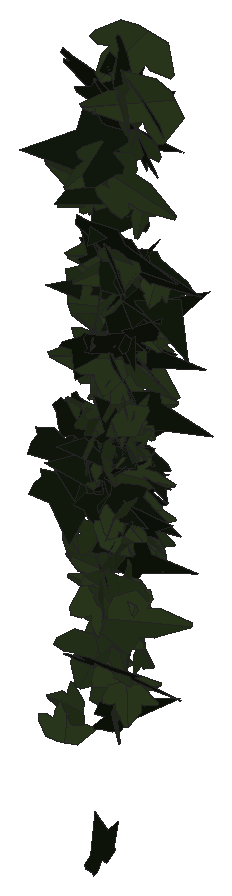
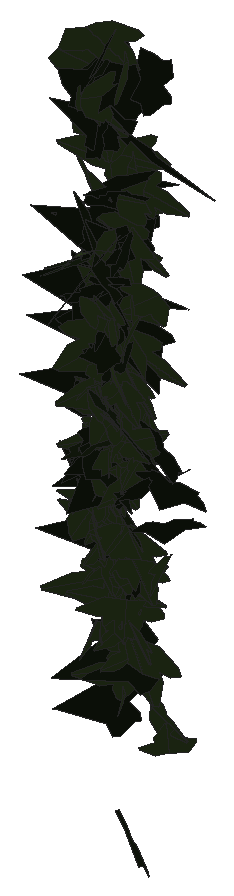
# SketchUp Ruby script. Lengths in inches.
U = 1.inch
M = Sketchup.active_model
def pt(a) = Geom::Point3d.new(a.map { |v| v * U })
def face(e, loops, mat)
  f = e.add_face(loops[0].map { |a| pt(a) })
  loops[1..].each { |l| e.add_face(l.map { |a| pt(a) }).erase! }
  f.material = f.back_material = mat if mat
  f
end
# faces: each face lists its corners as indices into pts; further lists are holes
def faces(e, pts, list, mat = nil) = list.each { |f| face(e, (f[0].is_a?(Array) ? f : [f]).map { |l| l.map { |i| pts[i] } }, mat) }
# xy, xz, yz: faces in a plane at the given z, y or x. An outline is a flat list of corners, or four numbers for a rectangle; further outlines are holes
def ring(l) = l.size == 4 ? [[l[0], l[1]], [l[2], l[1]], [l[2], l[3]], [l[0], l[3]]] : l.each_slice(2).to_a
def flat(e, list, mat, &to3) = list.each { |f| face(e, (f[0].is_a?(Array) ? f : [f]).map { |l| ring(l).map { |u, v| to3.(u, v) } }, mat) }
def xy(e, z, list, mat = nil) = flat(e, list, mat) { |x, y| [x, y, z] }
def xz(e, y, list, mat = nil) = flat(e, list, mat) { |x, z| [x, y, z] }
def yz(e, x, list, mat = nil) = flat(e, list, mat) { |y, z| [x, y, z] }
def lines(e, pts, list) = list.each { |a, b| e.add_line(pt(pts[a]), pt(pts[b])) }
# prism: a flat outline (further loops are holes) pulled along v
def prism(e, loops, v, mat = nil)
  f = face(e, loops, mat); d = Geom::Vector3d.new(v.map { |x| x * U })
  f.pushpull(f.normal.samedirection?(d) ? d.length : -d.length)
end
def box(e, o, s, mat = nil) = prism(e, [[o, [o[0] + s[0], o[1], o[2]], [o[0] + s[0], o[1] + s[1], o[2]], [o[0], o[1] + s[1], o[2]]]], [0, 0, s[2]], mat)
def at(x, y, z, deg = 0) = Geom::Transformation.translation(pt([x, y, z])) * Geom::Transformation.rotation(ORIGIN, Z_AXIS, deg.degrees)
def axes(o, x, y, z) = Geom::Transformation.new([*x, 0, *y, 0, *z, 0, *pt(o).to_a, 1])
def part(name) = M.definitions.add(name)
# library, detail: a bought-in or finely detailed component or shape, given as its bounding box
def library(name, o, s) = part(name).tap { |d| box(d.entities, o, s) }
def detail(e, o, s) = box(e.add_group.entities, o, s)
def put(e, d, t, mat = nil) = e.add_instance(d, t).tap { |i| i.material = mat if mat }
def group(e, t, mat = nil) = e.add_group.tap { |g| g.transformation = t; g.material = mat if mat }.entities
root = M.entities
M.materials.add("1026 AP 7946 SUNNY SIDE UP").color = [254, 231, 186]
M.materials.add("efeu1").color = [18, 25, 13]
M.materials.add("efeu2").color = [43, 57, 29]
c1 = part("ivyleaf_10")
p = [[0,0.5,-0.03],[-0.0625,2.02,-0.43],[-0.19,2.01,-0.46],[-0.54,1.05,-0.29],[-0.52,0.625,-0.18],[-0.83,0.76,-0.28],
  [-1.16,0.64,-0.33],[-1.15,0.33,-0.24],[-0.77,-0.39,0.02],[-0.3,-0.51,0.16],[0.04,-0.48,0.23],[-0.02,2.01,-0.4375],
  [-0.06,2.01,-0.43],[0.04,-0.49,0.23],[0.67,-0.49,0.14],[1.38,0.36,-0.2],[1.375,0.51,-0.24],[0.81,0.65,-0.19],
  [0.62,0.59,-0.15],[0.6,1.09,-0.28],[0.5,1.23,-0.31]]
faces(c1.entities,p,[[0,1,2,3,4,5,6,7,8,9,10],[11,12,0,13,14,15,16,17,18,19,20]],"efeu2")
c2 = part("ivyleaf_9")
p = [[1.54,2.16,1.25],[1.36,2.04,1.19],[-0.21,0.99,0.68],[-0.71,1.11,0.82],[-0.85,0.86,0.67],[-0.8,0.17,0.21],
  [-0.9,-0.01,0.1],[-0.67,-0.16,-0.02],[-0.08,-0.08,-0.05],[-0.03,-0.6,-0.4],[0.65,-0.88,-0.66],[0.83,-0.6,-0.49],
  [1.29,-0.42,-0.43],[1.8125,-0.07,-0.26],[1.21,0.44,0.15]]
faces(c2.entities,p,[[0,1,2,3,4,5,6,7,8,9,10,11,12,13,14]],"efeu1")
put(root,c1,axes([137.62,209.9,263.875],[0.11766,-0.06862,-0.22002],[0.29984,-0.09834,0.10099],[-0.18465,-0.2034,0.0238]),"1026 AP 7946 SUNNY SIDE UP")
put(root,c1,axes([138.34,209.98,262.02],[-0.01304,-0.02369,-0.22765],[0.16421,-0.19546,0.01642],[-0.30824,-0.10313,0.01838]),"1026 AP 7946 SUNNY SIDE UP")
put(root,c2,axes([138.23,209.71,261.3],[0.02182,-0.02112,-0.28857],[0.17202,0.25859,-0.01299],[0.40662,-0.10826,0.02098]),"1026 AP 7946 SUNNY SIDE UP")
put(root,c1,axes([138.18,209.91,258.03],[-0.11608,0.13996,-0.13331],[0.0679,-0.12375,-0.16299],[-0.2928,-0.08418,0.01505]),"1026 AP 7946 SUNNY SIDE UP")
put(root,c1,axes([137.95,210,266.1],[0.15276,0.12837,-0.25399],[-0.19782,-0.21344,-0.16632],[-0.39088,0.15819,-0.01509]),"1026 AP 7946 SUNNY SIDE UP")
put(root,c1,axes([138.28,209.68,261.9],[-0.08528,0.14601,0.20223],[-0.11746,0.18069,-0.15934],[-0.36522,-0.09221,0.00403]),"1026 AP 7946 SUNNY SIDE UP")
put(root,c1,axes([138.4375,209.86,258.39],[0.2544,0.13602,-0.00184],[0.01288,-0.0137,-0.21723],[-0.21353,0.16123,-0.01529]),"1026 AP 7946 SUNNY SIDE UP")
put(root,c2,axes([137.89,209.875,264.94],[0.34828,-0.08327,0.22073],[0.29953,-0.10121,-0.24345],[0.20355,0.29142,-0.01943]),"1026 AP 7946 SUNNY SIDE UP")
put(root,c2,axes([138.25,209.86,263.39],[0.43405,0.17022,0.04183],[-0.07626,0.00341,0.33286],[0.26403,-0.27885,0.02737]),"1026 AP 7946 SUNNY SIDE UP")
put(root,c1,axes([138.28,209.8,262.375],[0.43233,0.00207,0.1601],[-0.24322,0.03423,0.28167],[-0.02366,-0.31396,0.02991]),"1026 AP 7946 SUNNY SIDE UP")
put(root,c1,axes([138.3125,209.87,259.98],[-0.37139,-0.04498,0.01945],[-0.02256,-0.02646,-0.24669],[0.07348,-0.23548,0.02256]),"1026 AP 7946 SUNNY SIDE UP")
put(root,c1,axes([138.22,209.9,263.73],[-0.36976,-0.11445,-0.01028],[-0.02652,0.0134,0.26876],[-0.17859,0.23496,-0.01863]),"1026 AP 7946 SUNNY SIDE UP")
put(root,c2,axes([138.03,209.86,263.46],[0.12723,0.19476,-0.17816],[-0.08352,-0.16613,-0.21793],[-0.40213,0.09612,-0.01111]),"1026 AP 7946 SUNNY SIDE UP")
put(root,c1,axes([137.65,209.82,257.88],[-0.03585,0.04062,0.21877],[-0.3322,0.04013,-0.03107],[-0.07057,-0.20954,0.03514]),"1026 AP 7946 SUNNY SIDE UP")
put(root,c1,axes([138.34,209.99,262.51],[0.22732,-0.12361,0.12794],[0.12629,-0.09736,-0.19563],[0.24575,0.16438,-0.01781]),"1026 AP 7946 SUNNY SIDE UP")
put(root,c1,axes([138.04,209.9,259.81],[-0.03934,0.20759,-0.05095],[-0.03372,-0.05316,-0.21393],[-0.33429,-0.01907,0.02757]),"1026 AP 7946 SUNNY SIDE UP")
put(root,c1,axes([138.36,209.78,261.08],[0.12975,0.2141,0.14012],[0.07645,0.12573,-0.23564],[-0.39041,0.09578,0.00042]),"1026 AP 7946 SUNNY SIDE UP")
put(root,c1,axes([138.25,209.8,260.95],[0.06837,-0.1428,-0.14948],[-0.02841,0.14425,-0.15184],[0.31794,0.0436,0.01858]),"1026 AP 7946 SUNNY SIDE UP")
put(root,c1,axes([138.27,209.85,260.4],[-0.01717,-0.19277,-0.08617],[0.02222,0.0818,-0.19822],[0.32898,-0.01559,0.00889]),"1026 AP 7946 SUNNY SIDE UP")
put(root,c2,axes([138.35,209.95,260.96],[0.34035,-0.0054,-0.13599],[0.20697,0.02982,0.22132],[0.01722,-0.25175,0.02764]),"1026 AP 7946 SUNNY SIDE UP")
put(root,c1,axes([138.39,209.78,260.64],[0.1623,0.23022,-0.11099],[0.05265,0.10437,0.26027],[0.39707,-0.10794,0.01085]),"1026 AP 7946 SUNNY SIDE UP")
put(root,c1,axes([137.4375,209.82,257.46],[0.23002,0.16719,-0.0549],[0.03486,0.05245,0.22847],[0.27417,-0.14694,0.01701]),"1026 AP 7946 SUNNY SIDE UP")
put(root,c1,axes([138.26,210.07,264.625],[0.11058,0.08861,-0.29481],[-0.29876,-0.21474,-0.11765],[-0.36516,0.20252,0.00698]),"1026 AP 7946 SUNNY SIDE UP")
put(root,c1,axes([138.27,209.99,261.29],[-0.19135,-0.18041,0.12846],[-0.09051,-0.11254,-0.22443],[0.3337,-0.13397,0.01279]),"1026 AP 7946 SUNNY SIDE UP")
put(root,c1,axes([138.07,209.89,263.22],[0.22008,-0.0723,-0.28753],[-0.42865,0.06643,-0.15841],[0.14567,0.30471,-0.03172]),"1026 AP 7946 SUNNY SIDE UP")
put(root,c2,axes([138.45,210,262.16],[0.14585,0.0591,0.25072],[-0.36132,-0.08224,0.11047],[0.15533,-0.24679,0.02155]),"1026 AP 7946 SUNNY SIDE UP")
put(root,c1,axes([137.98,209.86,262.15],[-0.04842,-0.20496,0.10238],[0.01741,0.1,0.21407],[-0.35855,0.03253,-0.00343]),"1026 AP 7946 SUNNY SIDE UP")
put(root,c1,axes([138.1,210.02,267.41],[-0.22712,0.22157,-0.23308],[0.15552,-0.20612,-0.27269],[-0.47452,-0.1736,0.02219]),"1026 AP 7946 SUNNY SIDE UP")
put(root,c1,axes([138.8125,209.99,267.26],[0.27411,-0.00345,-0.33382],[-0.50519,-0.04968,-0.17782],[-0.06625,0.36457,-0.02522]),"1026 AP 7946 SUNNY SIDE UP")
put(root,c1,axes([138.3,209.89,264.85],[0.26794,-0.0938,-0.27633],[-0.40019,0.08733,-0.19791],[0.19693,0.30508,-0.02621]),"1026 AP 7946 SUNNY SIDE UP")
put(root,c2,axes([138.39,209.9,261.96],[-0.3289,0.14447,0.11019],[-0.16399,0.03459,-0.26004],[-0.22926,-0.23199,0.02793]),"1026 AP 7946 SUNNY SIDE UP")
put(root,c1,axes([137.86,210.09,265.48],[-0.03464,-0.0343,0.24621],[-0.13683,-0.22294,-0.0425],[0.35446,-0.08942,0.00766]),"1026 AP 7946 SUNNY SIDE UP")
put(root,c1,axes([138.48,209.73,259.5625],[-0.05382,-0.07102,-0.35717],[0.41431,0.22682,-0.07342],[0.37057,-0.26391,0.03021]),"1026 AP 7946 SUNNY SIDE UP")
put(root,c1,axes([138.13,209.92,262.52],[-0.30391,0.08898,-0.04726],[0.05561,-0.03379,-0.21881],[-0.14766,-0.19587,0.01486]),"1026 AP 7946 SUNNY SIDE UP")
put(root,c1,axes([138.46,209.82,261.68],[-0.09617,-0.05671,-0.23973],[0.31171,0.12221,-0.08376],[0.21049,-0.20689,0.01451]),"1026 AP 7946 SUNNY SIDE UP")
put(root,c1,axes([138.12,209.95,265.9],[0.08261,0.03072,0.37081],[0.56592,0.02478,-0.05618],[-0.04566,0.36274,-0.02542]),"1026 AP 7946 SUNNY SIDE UP")
put(root,c2,axes([138.22,209.99,264.74],[0.26101,-0.1018,0.26469],[0.3372,-0.14267,-0.20135],[0.27544,0.27112,-0.00432]),"1026 AP 7946 SUNNY SIDE UP")
put(root,c2,axes([137.89,209.79,258.68],[0.51816,-0.00778,0.08323],[0.12585,0.08835,-0.32684],[-0.02163,0.3276,0.09218]),"1026 AP 7946 SUNNY SIDE UP")
put(root,c2,axes([137.85,210.09,259.77],[-0.03768,-0.00594,0.24814],[0.02936,-0.24141,-0.00563],[0.37778,0.01817,0.02519]),"1026 AP 7946 SUNNY SIDE UP")
put(root,c1,axes([138.44,210.09,259.84],[-0.15714,-0.09343,0.15565],[0.15159,-0.17457,-0.04637],[0.23546,0.05003,0.13373]),"1026 AP 7946 SUNNY SIDE UP")
put(root,c1,axes([138.54,209.9,261.23],[-0.07983,-0.20533,-0.07381],[0.03525,0.06704,-0.21744],[0.33953,-0.05523,0.00522]),"1026 AP 7946 SUNNY SIDE UP")
put(root,c2,axes([138.31,209.77,260.71],[-0.08724,0.18956,0.18302],[-0.08976,0.1672,-0.20241],[-0.39734,-0.07939,0.00554]),"1026 AP 7946 SUNNY SIDE UP")
put(root,c1,axes([138.34,209.8125,259.3],[-0.06909,-0.0426,0.23517],[0.18638,0.19596,0.06226],[-0.31443,0.12551,-0.01477]),"1026 AP 7946 SUNNY SIDE UP")
put(root,c1,axes([138.17,210.05,260.75],[-0.15109,0.04966,-0.20345],[0.16456,-0.17563,-0.09884],[-0.27518,-0.13229,0.0526]),"1026 AP 7946 SUNNY SIDE UP")
put(root,c2,axes([138.08,209.94,266.27],[-0.42862,0.15289,0.1432],[-0.21515,0.03697,-0.32009],[-0.24225,-0.30335,0.03091]),"1026 AP 7946 SUNNY SIDE UP")
put(root,c2,axes([137.99,210.05,261.88],[-0.36049,-0.03909,-0.20502],[0.31525,-0.00058,-0.23808],[0.04583,-0.30344,0.02506]),"1026 AP 7946 SUNNY SIDE UP")
put(root,c1,axes([137.79,210.17,263.78],[-0.01479,0.13256,-0.33305],[0.04231,-0.32292,-0.13879],[-0.54888,-0.02846,-0.00172]),"1026 AP 7946 SUNNY SIDE UP")
put(root,c1,axes([138.32,210.03,259.125],[0.03956,-0.21025,0.07734],[0.11555,-0.06472,-0.20915],[0.33215,0.04756,0.06354]),"1026 AP 7946 SUNNY SIDE UP")
put(root,c1,axes([138.39,210.11,262.46],[0.00989,-0.16493,0.18574],[0.01953,-0.18085,-0.17105],[0.38482,0.01341,0.00391]),"1026 AP 7946 SUNNY SIDE UP")
put(root,c1,axes([137.87,209.9375,258.79],[0.51065,-0.0235,-0.08446],[-0.11609,0.08313,-0.32587],[0.06673,0.32443,0.07942]),"1026 AP 7946 SUNNY SIDE UP")
put(root,c2,axes([137.45,210.01,267.31],[0.3407,-0.12689,0.12004],[0.13743,-0.0817,-0.25798],[0.23432,0.23242,-0.02322]),"1026 AP 7946 SUNNY SIDE UP")
put(root,c1,axes([138.27,209.95,261.98],[-0.25696,-0.0733,0.13413],[0.17874,0.06519,0.18458],[-0.15336,0.19879,-0.00962]),"1026 AP 7946 SUNNY SIDE UP")
put(root,c1,axes([138.31,209.93,264.02],[0.2704,0.11295,0.193],[0.27766,0.06761,-0.2093],[-0.20156,0.24466,-0.02941]),"1026 AP 7946 SUNNY SIDE UP")
put(root,c1,axes([138.32,209.99,261.26],[0.36207,0.08113,0.03768],[0.06538,-0.00982,-0.25047],[-0.12338,0.23288,-0.02215]),"1026 AP 7946 SUNNY SIDE UP")
put(root,c2,axes([138.1,209.76,255.85],[-0.00882,0.11994,0.26245],[-0.0471,0.25242,-0.12196],[-0.43927,-0.02947,0.00781]),"1026 AP 7946 SUNNY SIDE UP")
put(root,c2,axes([138.27,209.77,261.52],[0.19699,0.14143,0.195],[0.20015,0.13903,-0.19382],[-0.31182,0.17859,-0.00122]),"1026 AP 7946 SUNNY SIDE UP")
put(root,c2,axes([138.2,210.01,264.54],[0.20309,-0.00299,0.23377],[-0.34488,0.06547,0.12987],[-0.09173,-0.25278,0.0293]),"1026 AP 7946 SUNNY SIDE UP")
put(root,c2,axes([138.33,209.89,260.33],[0.23259,0.04265,0.19869],[0.30494,0.01278,-0.15626],[-0.05697,0.24253,-0.02524]),"1026 AP 7946 SUNNY SIDE UP")
put(root,c2,axes([138.13,210.12,263.96],[-0.13517,-0.03774,-0.29123],[0.44373,-0.05248,-0.08156],[-0.06258,-0.29057,0.05077]),"1026 AP 7946 SUNNY SIDE UP")
put(root,c2,axes([138.04,210.17,263.01],[0.25668,-0.19461,-0.13537],[0.20571,-0.05596,0.25463],[-0.30544,-0.20123,0.05773]),"1026 AP 7946 SUNNY SIDE UP")
put(root,c2,axes([138.2,209.99,264.24],[0.0448,0.29861,0.20438],[-0.03877,-0.1952,0.30784],[0.56091,-0.03735,0.00496]),"1026 AP 7946 SUNNY SIDE UP")
put(root,c2,axes([137.29,210.1,260.94],[-0.15483,-0.22043,-0.04546],[0.05587,0.03093,-0.24772],[0.34865,-0.10284,0.01951]),"1026 AP 7946 SUNNY SIDE UP")
put(root,c1,axes([138.15,209.94,264.77],[-0.44333,0.08386,0.14589],[-0.22729,0.00618,-0.30122],[-0.1224,-0.31524,0.03093]),"1026 AP 7946 SUNNY SIDE UP")
put(root,c1,axes([138.28,209.91,259.56],[-0.23806,0.11866,0.1372],[-0.1876,0.0613,-0.19664],[-0.20743,-0.19163,0.02039]),"1026 AP 7946 SUNNY SIDE UP")
put(root,c2,axes([138.09,209.93,264.82],[0.33839,-0.15871,-0.20018],[-0.27838,0.08367,-0.27317],[0.27798,0.27699,-0.02988]),"1026 AP 7946 SUNNY SIDE UP")
put(root,c1,axes([138.4375,209.82,260.65],[-0.03347,-0.13974,-0.26517],[0.07982,0.2516,-0.14402],[0.45245,-0.05473,0.00579]),"1026 AP 7946 SUNNY SIDE UP")
put(root,c1,axes([137.875,210.11,259.9],[-0.11093,-0.07442,-0.195],[-0.24925,-0.1047,0.10289],[-0.19938,0.17229,-0.02013]),"1026 AP 7946 SUNNY SIDE UP")
put(root,c1,axes([138.1,209.83,258.39],[-0.00387,-0.02992,-0.30229],[0.33409,0.20311,-0.022],[0.32131,-0.21155,0.01923]),"1026 AP 7946 SUNNY SIDE UP")
put(root,c1,axes([138.1,210.05,261.1],[0.07641,0.18361,-0.077],[-0.03115,-0.07315,-0.19609],[-0.31077,0.05248,0.00072]),"1026 AP 7946 SUNNY SIDE UP")
put(root,c1,axes([138.33,210.08,263.65],[0.08792,-0.08688,-0.26225],[0.3545,-0.12578,0.09469],[-0.22934,-0.22773,0.04582]),"1026 AP 7946 SUNNY SIDE UP")
put(root,c2,axes([138.18,210.16,265.48],[-0.29985,-0.15689,0.02758],[-0.01464,-0.0321,-0.25385],[0.25008,-0.19,0.01821]),"1026 AP 7946 SUNNY SIDE UP")
put(root,c1,axes([138.51,210.1,265.65],[0.30391,-0.11855,0.08998],[0.09844,-0.0655,-0.23291],[0.21026,0.20202,-0.021]),"1026 AP 7946 SUNNY SIDE UP")
put(root,c1,axes([138.28,210.01,261.97],[-0.30122,0.07703,-0.03644],[0.03895,-0.03386,-0.21171],[-0.12776,-0.19193,0.02138]),"1026 AP 7946 SUNNY SIDE UP")
put(root,c1,axes([137.76,210.01,261.89],[-0.274,0.12532,-0.00599],[0.00578,0.01625,0.22065],[0.19723,0.17362,-0.01478]),"1026 AP 7946 SUNNY SIDE UP")
put(root,c1,axes([138.01,209.85,261.44],[0.04578,0.03449,-0.21689],[0.09952,0.20173,0.0442],[0.32067,-0.06753,0.01725]),"1026 AP 7946 SUNNY SIDE UP")
put(root,c1,axes([137.84,209.95,265.67],[0.03754,-0.03136,-0.30613],[-0.41808,0.13341,-0.03576],[0.21379,0.2664,-0.01616]),"1026 AP 7946 SUNNY SIDE UP")
put(root,c1,axes([138.31,210.06,262.39],[0.21701,-0.15909,-0.10224],[0.13087,-0.05721,0.21534],[-0.26337,-0.15951,0.02276]),"1026 AP 7946 SUNNY SIDE UP")
put(root,c1,axes([138.45,210.18,263.88],[0.00966,-0.17368,0.19789],[0.0038,-0.19308,-0.18014],[0.40833,0.0059,-0.003]),"1026 AP 7946 SUNNY SIDE UP")
put(root,c1,axes([138.13,209.99,262.31],[-0.44417,-0.11462,-0.10655],[0.168,0.00867,-0.31243],[0.17429,-0.30047,0.02962]),"1026 AP 7946 SUNNY SIDE UP")
put(root,c1,axes([138.32,210.18,260.59],[0.0107,-0.09234,0.20346],[0.0084,-0.19799,-0.09646],[0.34345,0.00772,-0.00398]),"1026 AP 7946 SUNNY SIDE UP")
put(root,c1,axes([138.05,210.03,259.66],[0.02874,0.04165,0.2225],[-0.33672,-0.04511,0.02739],[0.07738,-0.21177,0.03658]),"1026 AP 7946 SUNNY SIDE UP")
put(root,c2,axes([137.79,210.21,261.27],[-0.00328,-0.2101,-0.14011],[-0.00463,-0.13478,0.21566],[-0.39249,0.00335,-0.00137]),"1026 AP 7946 SUNNY SIDE UP")
put(root,c2,axes([138.55,209.77,263.84],[0.04352,0.06541,0.37256],[0.45369,0.22016,-0.06255],[-0.35699,0.28777,-0.03408]),"1026 AP 7946 SUNNY SIDE UP")
put(root,c1,axes([138.27,210.11,260.95],[-0.08727,-0.18019,0.09732],[-0.02357,-0.09509,-0.19439],[0.31979,-0.05618,0.01223]),"1026 AP 7946 SUNNY SIDE UP")
put(root,c1,axes([138.22,209.88,262.33],[-0.05709,0.0677,0.24194],[-0.24945,0.17358,-0.07593],[-0.29159,-0.16174,0.01759]),"1026 AP 7946 SUNNY SIDE UP")
put(root,c1,axes([138.04,209.87,258.625],[0.00881,0.02645,0.21993],[-0.00199,0.21341,-0.02598],[-0.33801,-0.00056,0.00588]),"1026 AP 7946 SUNNY SIDE UP")
put(root,c1,axes([137.89,210.15,261.96],[0.10653,0.12988,-0.17475],[-0.11278,-0.15462,-0.15173],[-0.31742,0.09853,-0.00474]),"1026 AP 7946 SUNNY SIDE UP")
put(root,c1,axes([138.43,210.19,262.57],[-0.18301,-0.11755,0.15174],[0.15475,-0.18605,-0.07361],[0.25366,0.02869,0.15439]),"1026 AP 7946 SUNNY SIDE UP")
put(root,c1,axes([138.41,210.1,260.875],[-0.16246,0.06512,-0.20116],[0.24196,-0.1213,-0.12602],[-0.2158,-0.18503,0.01014]),"1026 AP 7946 SUNNY SIDE UP")
put(root,c1,axes([137.88,210.05,260.43],[-0.35193,-0.0185,0.11804],[-0.17237,-0.04873,-0.22879],[0.06043,-0.24672,0.03483]),"1026 AP 7946 SUNNY SIDE UP")
put(root,c1,axes([137.79,210.08,259.18],[0.2324,-0.15923,-0.00879],[-0.02482,-0.00426,-0.22334],[0.24942,0.14793,-0.01403]),"1026 AP 7946 SUNNY SIDE UP")
put(root,c2,axes([138.375,209.875,261.75],[0.00847,-0.04135,-0.28042],[-0.10223,0.26412,-0.04115],[0.4203,0.06508,-0.00436]),"1026 AP 7946 SUNNY SIDE UP")
put(root,c2,axes([138.27,210.17,264.1],[-0.11981,-0.12524,-0.24098],[-0.23987,-0.17756,0.14854],[-0.34017,0.16931,-0.01987]),"1026 AP 7946 SUNNY SIDE UP")
put(root,c2,axes([138.04,210.29,265.74],[-0.29708,-0.15379,0.199],[-0.19353,-0.15345,-0.24965],[0.33781,-0.22316,0.03198]),"1026 AP 7946 SUNNY SIDE UP")
put(root,c2,axes([137.2,210.12,261.58],[-0.23559,-0.10264,-0.16764],[0.23244,0.06943,-0.1856],[0.19239,-0.20957,0.01896]),"1026 AP 7946 SUNNY SIDE UP")
put(root,c1,axes([138.64,210.22,264.45],[-0.21772,-0.0851,0.16648],[0.1546,-0.206,-0.0261],[0.24282,0.05485,0.16589]),"1026 AP 7946 SUNNY SIDE UP")
put(root,c2,axes([138.39,210.21,267.2],[0.11169,-0.19126,0.14792],[0.0666,-0.13851,-0.21087],[0.37115,0.08241,-0.00667]),"1026 AP 7946 SUNNY SIDE UP")
put(root,c2,axes([138.37,210,263.375],[0.22765,0.00596,0.20507],[0.31262,-0.01789,-0.14854],[0.01726,0.24546,-0.01436]),"1026 AP 7946 SUNNY SIDE UP")
put(root,c1,axes([138.09,210,261.73],[-0.10629,0.19021,0.06336],[-0.08827,0.0431,-0.20421],[-0.30114,-0.07977,0.0375]),"1026 AP 7946 SUNNY SIDE UP")
put(root,c1,axes([138.08,209.97,259.09],[-0.06036,-0.13011,-0.17232],[0.16664,0.13459,-0.13271],[0.2875,-0.10533,0.04074]),"1026 AP 7946 SUNNY SIDE UP")
put(root,c2,axes([138.1875,210.27,267.625],[0.10445,-0.1068,-0.2385],[0.24808,-0.16992,0.12673],[-0.31381,-0.16987,0.0208]),"1026 AP 7946 SUNNY SIDE UP")
put(root,c1,axes([138.04,210.18,262.8125],[0.11599,0.10246,-0.18029],[-0.15682,-0.14453,-0.13089],[-0.27855,0.12403,-0.00138]),"1026 AP 7946 SUNNY SIDE UP")
put(root,c1,axes([138.08,210.08,263.56],[-0.00798,-0.22254,-0.02854],[-0.00544,0.02652,-0.22912],[0.35234,-0.00463,-0.00419]),"1026 AP 7946 SUNNY SIDE UP")
put(root,c2,axes([138.36,210.22,264.56],[0.07052,-0.40224,-0.03228],[0.14715,0.03881,-0.40456],[0.61682,0.03673,0.1002]),"1026 AP 7946 SUNNY SIDE UP")
put(root,c1,axes([138.28,210.07,262.51],[0.22637,0.07973,0.14082],[0.2108,0.0356,-0.16719],[-0.13105,0.19499,-0.02568]),"1026 AP 7946 SUNNY SIDE UP")
put(root,c2,axes([137.28,210.17,262.09],[-0.06008,-0.05158,-0.25654],[0.39766,0.01585,-0.04332],[0.03743,-0.25114,0.04842]),"1026 AP 7946 SUNNY SIDE UP")
put(root,c1,axes([138.29,210.05,263.74],[-0.29434,0.10521,0.09923],[-0.1607,0.01056,-0.21778],[-0.15556,-0.20998,0.03723]),"1026 AP 7946 SUNNY SIDE UP")
put(root,c1,axes([137.92,210.11,259.5],[0.39651,0.21819,0.00123],[0.02482,-0.01832,-0.34273],[-0.34218,0.2515,-0.02344]),"1026 AP 7946 SUNNY SIDE UP")
put(root,c2,axes([138.43,210.01,262.4],[-0.21317,0.22662,0.066],[-0.07079,0.04611,-0.27136],[-0.36291,-0.14211,0.01417]),"1026 AP 7946 SUNNY SIDE UP")
put(root,c1,axes([137.54,210.11,264.18],[-0.27607,-0.00274,-0.15324],[0.22971,-0.04659,-0.17704],[-0.04413,-0.22534,0.0371]),"1026 AP 7946 SUNNY SIDE UP")
put(root,c2,axes([138.12,209.875,257.93],[0.16653,0.10718,0.27248],[0.31481,0.17223,-0.15384],[-0.31853,0.22625,-0.00959]),"1026 AP 7946 SUNNY SIDE UP")
put(root,c2,axes([138.4,210.02,262.5625],[0.15369,0.02417,-0.2552],[0.26004,0.19277,0.08768],[0.29276,-0.18391,0.05609]),"1026 AP 7946 SUNNY SIDE UP")
put(root,c1,axes([137.36,210.02,260.31],[-0.05826,0.21091,0.08241],[-0.02745,0.07692,-0.22012],[-0.35295,-0.0408,0.00352]),"1026 AP 7946 SUNNY SIDE UP")
put(root,c1,axes([137.99,210.16,261.33],[0.04644,0.2072,-0.10364],[-0.04635,-0.09838,-0.21573],[-0.36002,0.03939,0.01441]),"1026 AP 7946 SUNNY SIDE UP")
put(root,c1,axes([138.2,210.04,263.3125],[-0.40898,-0.11655,-0.25021],[0.38179,0.04273,-0.28953],[0.18133,-0.35284,0.04526]),"1026 AP 7946 SUNNY SIDE UP")
put(root,c1,axes([138.37,209.94,262.48],[-0.01882,0.02645,-0.2366],[-0.07874,0.22437,0.0306],[0.35512,0.05115,-0.00575]),"1026 AP 7946 SUNNY SIDE UP")
put(root,c1,axes([138.41,210.15,266.97],[-0.15204,-0.22782,0.0313],[-0.00674,-0.03257,-0.255],[0.36161,-0.0964,0.00841]),"1026 AP 7946 SUNNY SIDE UP")
put(root,c1,axes([138.26,210.33,266.97],[-0.05019,-0.00202,0.30622],[-0.04364,-0.29764,-0.00689],[0.46538,-0.02813,0.03238]),"1026 AP 7946 SUNNY SIDE UP")
put(root,c1,axes([138.34,210.08,261.98],[-0.16586,0.07256,0.18492],[-0.30019,-0.00763,-0.1127],[-0.04691,-0.2077,0.06738]),"1026 AP 7946 SUNNY SIDE UP")
put(root,c1,axes([138.11,210.13,263.02],[0.09656,-0.23216,-0.02528],[-0.02809,0.01926,-0.24696],[0.3658,0.06276,-0.01229]),"1026 AP 7946 SUNNY SIDE UP")
put(root,c1,axes([138.49,210.05,258.95],[0.07349,-0.16739,-0.11616],[0.0903,0.1211,-0.16134],[0.30337,0.0045,0.07616]),"1026 AP 7946 SUNNY SIDE UP")
put(root,c2,axes([138.12,210.1875,266.91],[0.39702,0.05244,0.19979],[-0.3083,-0.00141,0.26376],[0.06679,-0.31819,0.02985]),"1026 AP 7946 SUNNY SIDE UP")
put(root,c2,axes([138.35,210.1,261.6],[-0.10675,0.22389,-0.08737],[0.02851,-0.08441,-0.24141],[-0.37608,-0.06995,0.0065]),"1026 AP 7946 SUNNY SIDE UP")
put(root,c2,axes([138.22,210.27,266.44],[0.13302,-0.04521,-0.2403],[0.35405,-0.06293,0.09643],[-0.118,-0.23976,0.01845]),"1026 AP 7946 SUNNY SIDE UP")
put(root,c2,axes([138.34,209.96,261.19],[0.18413,0.17823,0.12435],[0.12867,0.08899,-0.21847],[-0.3121,0.14184,-0.01671]),"1026 AP 7946 SUNNY SIDE UP")
put(root,c2,axes([138.375,210.08,264.45],[0.29123,-0.25403,-0.22682],[-0.20276,0.17668,-0.32285],[0.48656,0.22568,0.00123]),"1026 AP 7946 SUNNY SIDE UP")
put(root,c1,axes([138.32,210.24,267.87],[0.41163,0.12751,-0.18289],[-0.23088,-0.10412,-0.29948],[-0.25585,0.29911,-0.024]),"1026 AP 7946 SUNNY SIDE UP")
put(root,c2,axes([138.32,210.26,261.78],[0.04376,-0.24135,0.04676],[0.12553,-0.03563,-0.23864],[0.3656,0.04112,0.07634]),"1026 AP 7946 SUNNY SIDE UP")
put(root,c1,axes([138.39,210.13,266.52],[-0.36281,0.01606,0.08778],[-0.13578,-0.02345,-0.23672],[-0.01079,-0.24482,0.02699]),"1026 AP 7946 SUNNY SIDE UP")
put(root,c1,axes([138.39,210,260.24],[0.00598,-0.06754,-0.2157],[0.05959,0.20609,-0.0667],[0.34017,-0.03491,0.01548]),"1026 AP 7946 SUNNY SIDE UP")
put(root,c1,axes([138,210.15,262.68],[-0.29348,0.00868,0.11105],[-0.16942,-0.03206,-0.18982],[0.01353,-0.21311,0.03181]),"1026 AP 7946 SUNNY SIDE UP")
put(root,c2,axes([138.07,210.18,266.46],[0.14177,-0.06953,0.22129],[0.30077,-0.10015,-0.11648],[0.18971,0.21074,0.0193]),"1026 AP 7946 SUNNY SIDE UP")
put(root,c1,axes([138.25,210.09,261.59],[-0.01257,0.20011,0.05633],[-0.12378,0.04663,-0.19137],[-0.30129,-0.0275,0.07627]),"1026 AP 7946 SUNNY SIDE UP")
put(root,c1,axes([137.73,210.16,262.93],[0.25307,-0.14094,-0.0806],[-0.10064,0.04437,-0.21997],[0.23197,0.173,-0.0075]),"1026 AP 7946 SUNNY SIDE UP")
put(root,c2,axes([138.45,210.33,264.05],[-0.27117,-0.14981,0.10825],[-0.10464,-0.0844,-0.23508],[0.26885,-0.18395,0.01769]),"1026 AP 7946 SUNNY SIDE UP")
put(root,c1,axes([137.88,210.19,261.98],[-0.20278,-0.02375,-0.20856],[-0.31881,-0.00807,0.13407],[-0.03081,0.23978,-0.01473]),"1026 AP 7946 SUNNY SIDE UP")
put(root,c1,axes([138.3,209.93,262.62],[-0.06588,-0.093,-0.35398],[0.29262,0.28859,-0.10231],[0.4762,-0.1902,0.0139]),"1026 AP 7946 SUNNY SIDE UP")
put(root,c1,axes([138.375,210.14,260.59],[0.07067,-0.19737,-0.06935],[-0.03486,0.0628,-0.20804],[0.32548,0.04958,-0.00722]),"1026 AP 7946 SUNNY SIDE UP")
put(root,c1,axes([138.46,210.15,260.93],[0.26672,0.11588,0.07597],[0.11179,0.02498,-0.21064],[-0.18414,0.183,-0.01783]),"1026 AP 7946 SUNNY SIDE UP")
put(root,c1,axes([138.04,210.1,260.58],[0.13248,0.19683,0.08058],[0.04374,0.07195,-0.22013],[-0.3295,0.08869,0.00317]),"1026 AP 7946 SUNNY SIDE UP")
put(root,c1,axes([138.51,210.17,260.65],[0.32831,-0.01802,0.10664],[0.16528,0.02798,-0.21303],[0.00558,0.23141,0.03544]),"1026 AP 7946 SUNNY SIDE UP")
put(root,c2,axes([138.05,210.22,263.32],[0.27838,-0.14851,0.07656],[0.07626,-0.05895,-0.238],[0.25036,0.18308,-0.01264]),"1026 AP 7946 SUNNY SIDE UP")
put(root,c1,axes([137.7,210.15,260.17],[0.33081,0.05103,-0.07051],[-0.12479,0.04793,-0.21333],[-0.05044,0.21607,0.06536]),"1026 AP 7946 SUNNY SIDE UP")
put(root,c1,axes([137.77,210.05,261.61],[-0.03481,-0.1165,-0.17803],[0.06236,0.16757,-0.12111],[0.32084,-0.04521,0.00422]),"1026 AP 7946 SUNNY SIDE UP")
